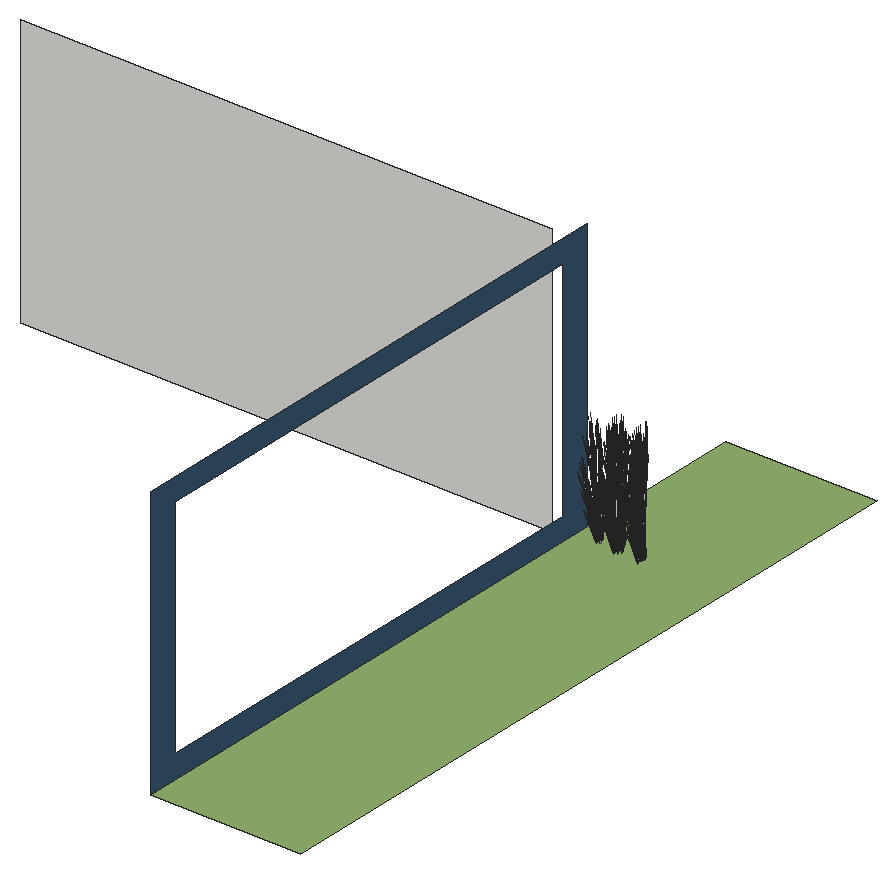
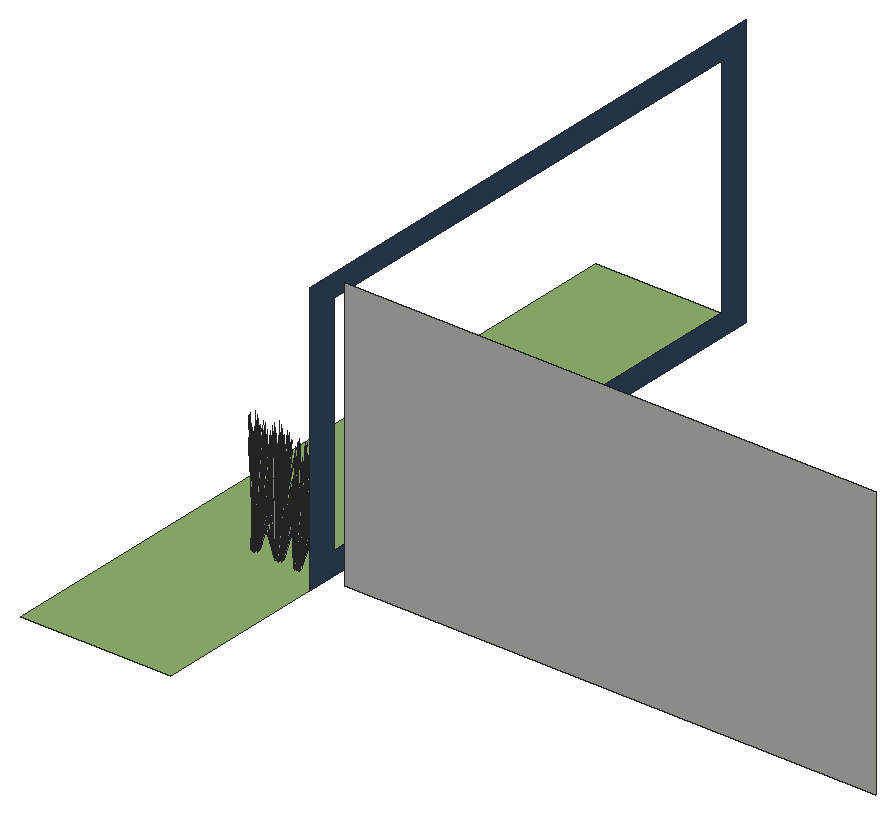
# SketchUp Ruby script. Lengths in inches.
U = 1.inch
M = Sketchup.active_model
def pt(a) = Geom::Point3d.new(a.map { |v| v * U })
def face(e, loops, mat)
  f = e.add_face(loops[0].map { |a| pt(a) })
  loops[1..].each { |l| e.add_face(l.map { |a| pt(a) }).erase! }
  f.material = f.back_material = mat if mat
  f
end
# faces: each face lists its corners as indices into pts; further lists are holes
def faces(e, pts, list, mat = nil) = list.each { |f| face(e, (f[0].is_a?(Array) ? f : [f]).map { |l| l.map { |i| pts[i] } }, mat) }
# xy, xz, yz: faces in a plane at the given z, y or x. An outline is a flat list of corners, or four numbers for a rectangle; further outlines are holes
def ring(l) = l.size == 4 ? [[l[0], l[1]], [l[2], l[1]], [l[2], l[3]], [l[0], l[3]]] : l.each_slice(2).to_a
def flat(e, list, mat, &to3) = list.each { |f| face(e, (f[0].is_a?(Array) ? f : [f]).map { |l| ring(l).map { |u, v| to3.(u, v) } }, mat) }
def xy(e, z, list, mat = nil) = flat(e, list, mat) { |x, y| [x, y, z] }
def xz(e, y, list, mat = nil) = flat(e, list, mat) { |x, z| [x, y, z] }
def yz(e, x, list, mat = nil) = flat(e, list, mat) { |y, z| [x, y, z] }
def lines(e, pts, list) = list.each { |a, b| e.add_line(pt(pts[a]), pt(pts[b])) }
# prism: a flat outline (further loops are holes) pulled along v
def prism(e, loops, v, mat = nil)
  f = face(e, loops, mat); d = Geom::Vector3d.new(v.map { |x| x * U })
  f.pushpull(f.normal.samedirection?(d) ? d.length : -d.length)
end
def box(e, o, s, mat = nil) = prism(e, [[o, [o[0] + s[0], o[1], o[2]], [o[0] + s[0], o[1] + s[1], o[2]], [o[0], o[1] + s[1], o[2]]]], [0, 0, s[2]], mat)
def at(x, y, z, deg = 0) = Geom::Transformation.translation(pt([x, y, z])) * Geom::Transformation.rotation(ORIGIN, Z_AXIS, deg.degrees)
def axes(o, x, y, z) = Geom::Transformation.new([*x, 0, *y, 0, *z, 0, *pt(o).to_a, 1])
def part(name) = M.definitions.add(name)
# library, detail: a bought-in or finely detailed component or shape, given as its bounding box
def library(name, o, s) = part(name).tap { |d| box(d.entities, o, s) }
def detail(e, o, s) = box(e.add_group.entities, o, s)
def put(e, d, t, mat = nil) = e.add_instance(d, t).tap { |i| i.material = mat if mat }
def group(e, t, mat = nil) = e.add_group.tap { |g| g.transformation = t; g.material = mat if mat }.entities
root = M.entities
M.materials.add("Carpet_04_1K").color = [56, 85, 112]
M.materials.add("LightPink_Translucent").color = [144, 107, 117]
M.materials["LightPink_Translucent"].alpha = 0.75
M.materials.add("Roofing_02_1K").color = [146, 178, 111]
c1 = part("blade")
p = [[2.15,0.21,22],[0,0.17,0],[0.09,0.45,0],[2.18,0.31,22],[2.29,0.31,22],[0.38,0.45,0],
  [2.48,0.24,33],[2.49,0.24,33],[2.48,0.22,33]]
faces(c1.entities,p,[[0,1,2,3],[4,5,2,3],[6,3,4,7],[8,0,3,6]])
c2 = part("seeds")
p = [[0.3,-0.1,1.38],[-0.01,-0.03,1.59],[-0.01,-0.03,0.03],[0.14,-0.07,-0.07],[0.29,-0.03,3],[0.15,0.01,3.11]]
faces(c2.entities,p,[[0,1,2,3],[1,0,4,5]],"LightPink_Translucent")
c3 = part("blade with seeds")
put(c3.entities,c1,at(0,0,0))
put(c3.entities,c2,axes([2.4,0.25,30.99],[1.5799,-0.05474,1.17369],[-0.12525,1.92788,0.29478],[-0.07173,-0.02425,1.56792]))
xy(root,0,[[330.57,509.26,410.57,890.67]],"Roofing_02_1K")
xz(root,786.64,[[39.57,0,321.57,144]])
yz(root,330.57,[[[509.26,0,798.7,144],[525.34,12,782.62,132]]],"Carpet_04_1K")
put(root,c3,axes([367.32,786.74,3.875],[0.08068,0.14973,1.71376],[-0.3728,0.12606,0.13857],[-0.08426,-0.23506,0.73262]))
put(root,c3,axes([368.3125,786.86,4.98],[-0.16845,-0.3792,-0.71045],[0.34676,-0.21133,0.08574],[-0.03939,-0.18322,1.00501]))
put(root,c3,axes([367.22,786.35,2.59],[-0.02137,0.15256,1.43002],[-0.31245,0.12771,-0.30754],[-0.07303,-0.19719,0.61141]))
put(root,c3,axes([354.24,787.1,3.875],[0.08068,0.14973,1.71376],[-0.3728,0.12606,0.13857],[-0.08426,-0.23506,0.73262]))
put(root,c3,axes([368.02,786.01,1.49],[-0.0592,0.0168,1.76342],[-0.32738,-0.18913,-0.26939],[0.00549,-0.15776,0.30037]))
put(root,c3,axes([355.69,786.88,2.59],[-0.10032,0.0944,1.43002],[-0.30046,-0.16522,-0.30754],[0.05569,-0.20547,0.61141]))
put(root,c3,axes([355.23,787.21,4.98],[-0.16845,-0.3792,-0.71045],[0.34676,-0.21133,0.08574],[-0.03939,-0.18322,1.00501]))
put(root,c3,axes([354.14,786.7,2.59],[-0.02137,0.15256,1.43002],[-0.31245,0.12771,-0.30754],[-0.07303,-0.19719,0.61141]))
put(root,c3,axes([368.34,786.53,4.53],[0.1064,-0.35863,-0.35414],[0.31043,0.1046,0.4572],[-0.02846,-0.14439,0.87481]))
put(root,c3,axes([354.94,786.37,1.49],[-0.0592,0.0168,1.76342],[-0.32738,-0.18913,-0.26939],[0.00549,-0.15776,0.30037]))
put(root,c3,axes([368.1875,786.78,4.68],[-0.34695,-0.11691,-0.51099],[0.11892,-0.40083,-0.3958],[-0.03181,-0.16138,0.97773]))
put(root,c3,axes([368.4,785.78,2.77],[0.04528,0.27194,1.1486],[-0.25117,-0.15062,0.84392],[0.02703,-0.13924,0.25299]))
put(root,c3,axes([355.93,787.58,4.98],[0.00918,-0.43138,-0.71045],[0.38672,0.02897,0.08574],[0.04081,-0.18275,1.00501]))
put(root,c3,axes([368.9375,787.08,4.68],[-0.25266,-0.31335,-0.51099],[0.2669,-0.27442,-0.3958],[0.03844,-0.15921,0.97773]))
put(root,c3,axes([355.27,786.89,4.53],[0.1064,-0.35863,-0.35414],[0.31043,0.1046,0.4572],[-0.02846,-0.14439,0.87481]))
put(root,c3,axes([355.5,787.36,3.875],[-0.06572,0.16029,1.71376],[-0.27569,-0.33172,0.13857],[0.12437,-0.20675,0.73262]))
put(root,c3,axes([355.11,787.13,4.68],[-0.34695,-0.11691,-0.51099],[0.11892,-0.40083,-0.3958],[-0.03181,-0.16138,0.97773]))
put(root,c3,axes([355.32,786.13,2.77],[0.04528,0.27194,1.1486],[-0.25117,-0.15062,0.84392],[0.02703,-0.13924,0.25299]))
put(root,c3,axes([355.86,787.4375,4.68],[-0.25266,-0.31335,-0.51099],[0.2669,-0.27442,-0.3958],[0.03844,-0.15921,0.97773]))
put(root,c3,axes([367.11,786.1,2.77],[0.18411,0.16231,1.1486],[-0.26813,0.09757,0.84392],[-0.05737,-0.12474,0.25299]))
put(root,c3,axes([367.55,786.96,4.98],[-0.30095,-0.22541,-0.71045],[0.21388,-0.395,0.08574],[-0.10904,-0.13459,1.00501]))
put(root,c3,axes([367.45,786.66,4.53],[-0.05451,-0.37564,-0.35414],[0.31161,-0.09919,0.4572],[-0.0837,-0.10765,0.87481]))
put(root,c3,axes([356.09,787.32,4.53],[0.23881,-0.24554,-0.35414],[0.22606,0.28036,0.4572],[0.0344,-0.14245,0.87481]))
put(root,c3,axes([354.03,786.46,2.77],[0.18411,0.16231,1.1486],[-0.26813,0.09757,0.84392],[-0.05737,-0.12474,0.25299]))
put(root,c3,axes([354.47,787.32,4.98],[-0.30095,-0.22541,-0.71045],[0.21388,-0.395,0.08574],[-0.10904,-0.13459,1.00501]))
put(root,c3,axes([354.37,787.02,4.53],[-0.05451,-0.37564,-0.35414],[0.31161,-0.09919,0.4572],[-0.0837,-0.10765,0.87481]))
put(root,c3,axes([366.96,786.59,1.49],[-0.03419,0.06144,1.76342],[-0.3455,0.13246,-0.26939],[-0.08346,-0.12049,0.30037]))
put(root,c3,axes([367.53,788.28,2.1],[-0.14494,-0.47823,-0.69835],[0.41752,-0.17223,-0.18329],[-0.01602,-0.16194,1.54149]))
put(root,c3,axes([366.78,787.21,3.875],[0.1311,0.08035,1.71376],[-0.27131,0.33708,0.13857],[-0.16909,-0.15206,0.73262]))
put(root,c3,axes([367.41,786.97,4.68],[-0.34827,0.11086,-0.51099],[-0.06092,-0.41983,-0.3958],[-0.09354,-0.12031,0.97773]))
put(root,c3,axes([353.88,786.95,1.49],[-0.03419,0.06144,1.76342],[-0.3455,0.13246,-0.26939],[-0.08346,-0.12049,0.30037]))
put(root,c3,axes([354.45,788.63,2.1],[-0.14494,-0.47823,-0.69835],[0.41752,-0.17223,-0.18329],[-0.01602,-0.16194,1.54149]))
put(root,c3,axes([353.7,787.57,3.875],[0.1311,0.08035,1.71376],[-0.27131,0.33708,0.13857],[-0.16909,-0.15206,0.73262]))
put(root,c3,axes([356.39,787.17,1.49],[-0.05283,-0.03674,1.76342],[-0.13569,-0.41045,-0.26939],[0.09154,-0.11138,0.30037]))
put(root,c3,axes([367.48,786.91,2.375],[-0.22066,-0.46731,0],[0.36918,-0.26061,-0.51607],[0.08408,-0.05936,1.63711]))
put(root,c3,axes([367.96,786.34,2.13],[-0.2439,0.26754,-0.03893],[-0.22348,-0.29302,-0.17649],[-0.01573,-0.08303,0.58215]))
put(root,c3,axes([354.33,787.33,4.68],[-0.34827,0.11086,-0.51099],[-0.06092,-0.41983,-0.3958],[-0.09354,-0.12031,0.97773]))
put(root,c3,axes([356.39,788.33,4.98],[0.18436,-0.36797,-0.71045],[0.32306,0.26151,0.08574],[0.11008,-0.13332,1.00501]))
put(root,c3,axes([354.4,787.26,2.375],[-0.22066,-0.46731,0],[0.36918,-0.26061,-0.51607],[0.08408,-0.05936,1.63711]))
put(root,c3,axes([356.38,788.16,4.68],[-0.09067,-0.42583,-0.51099],[0.34336,-0.07449,-0.3958],[0.0984,-0.11438,0.97773]))
put(root,c3,axes([354.88,786.7,2.13],[-0.2439,0.26754,-0.03893],[-0.22348,-0.29302,-0.17649],[-0.01573,-0.08303,0.58215]))
put(root,c3,axes([368.27,789.51,3.33],[0.305,0.18805,1.51261],[-0.29879,0.40513,0.59816],[-0.13384,-0.24012,1.26806]))
put(root,c3,axes([342.99,789.57,3.875],[0.08068,0.14973,1.71376],[-0.3728,0.12606,0.13857],[-0.08426,-0.23506,0.73262]))
put(root,c3,axes([366.68,788.21,2.02],[0,-0.46636,-0.49651],[0.39487,0,0],[0,-0.10622,1.57504]))
put(root,c3,axes([344.44,789.35,2.59],[-0.10032,0.0944,1.43002],[-0.30046,-0.16522,-0.30754],[0.05569,-0.20547,0.61141]))
put(root,c3,axes([343.98,789.68,4.98],[-0.16845,-0.3792,-0.71045],[0.34676,-0.21133,0.08574],[-0.03939,-0.18322,1.00501]))
put(root,c3,axes([342.89,789.18,2.59],[-0.02137,0.15256,1.43002],[-0.31245,0.12771,-0.30754],[-0.07303,-0.19719,0.61141]))
put(root,c3,axes([355.19,789.87,3.33],[0.305,0.18805,1.51261],[-0.29879,0.40513,0.59816],[-0.13384,-0.24012,1.26806]))
put(root,c3,axes([343.69,788.84,1.49],[-0.0592,0.0168,1.76342],[-0.32738,-0.18913,-0.26939],[0.00549,-0.15776,0.30037]))
put(root,c3,axes([353.6,788.57,2.02],[0,-0.46636,-0.49651],[0.39487,0,0],[0,-0.10622,1.57504]))
put(root,c3,axes([354.7,787.1875,2.02],[0.33032,-0.23318,-0.49651],[0.19744,0.41812,0],[0.07523,-0.05311,1.57504]))
put(root,c3,axes([356.66,787.99,2.59],[-0.12609,-0.01381,1.43002],[-0.12917,-0.37055,-0.30754],[0.1549,-0.10482,0.61141]))
put(root,c3,axes([367.75,788.4,2.21],[0.17124,-0.42022,-0.44739],[0.35581,0.20224,0.21531],[0,-0.09687,1.43643]))
put(root,c3,axes([366.73,787.33,4.53],[-0.20082,-0.29199,-0.35414],[0.2293,-0.2764,0.4572],[-0.1165,-0.04206,0.87481]))
put(root,c3,axes([355.09,788.14,2.06],[0.23773,-0.35053,-0.62353],[0.29532,0.31785,-0.16365],[0.09526,-0.08744,1.37633]))
put(root,c3,axes([344.68,790.05,4.98],[0.00918,-0.43138,-0.71045],[0.38672,0.02897,0.08574],[0.04081,-0.18275,1.00501]))
put(root,c3,axes([367.91,788.2,2.67],[-0.04113,-0.53214,-0.29095],[0.42835,-0.03218,-0.50002],[0.07543,-0.07088,1.59708]))
put(root,c3,axes([356.8,787.3125,2.77],[-0.11756,0.2374,1.1486],[-0.10105,-0.31895,0.84392],[0.09709,-0.07992,0.25299]))
put(root,c3,axes([366.85,788.22,2.03],[0.24637,-0.29097,-0.30978],[0.24637,0.29097,0.30978],[0,-0.09372,1.38974]))
put(root,c3,axes([366.75,786.83,2.13],[-0.10181,0.3808,-0.03893],[-0.31336,-0.11714,-0.17649],[-0.04758,-0.06228,0.58215]))
put(root,c3,axes([367.71,788.75,2.67],[-0.39748,-0.22252,-0.29095],[0.19139,-0.46966,-0.50002],[-0.01249,-0.11531,1.59708]))
put(root,c3,axes([344.01,789.36,4.53],[0.1064,-0.35863,-0.35414],[0.31043,0.1046,0.4572],[-0.02846,-0.14439,0.87481]))
put(root,c3,axes([344.25,789.83,3.875],[-0.06572,0.16029,1.71376],[-0.27569,-0.33172,0.13857],[0.12437,-0.20675,0.73262]))
put(root,c3,axes([366.58,788.57,2.375],[-0.44133,0,0],[0,-0.52122,-0.51607],[0,-0.11871,1.63711]))
put(root,c3,axes([356.63,788.2,4.53],[0.30722,-0.06665,-0.35414],[0.08112,0.381,0.4572],[0.08804,-0.10234,0.87481]))
put(root,c3,axes([366.66,787.64,2.59],[0.06891,0.12984,1.43002],[-0.15879,0.35293,-0.30754],[-0.16304,-0.08436,0.61141]))
put(root,c3,axes([343.86,789.61,4.68],[-0.34695,-0.11691,-0.51099],[0.11892,-0.40083,-0.3958],[-0.03181,-0.16138,0.97773]))
put(root,c3,axes([354.67,788.76,2.21],[0.17124,-0.42022,-0.44739],[0.35581,0.20224,0.21531],[0,-0.09687,1.43643]))
put(root,c3,axes([353.65,787.68,4.53],[-0.20082,-0.29199,-0.35414],[0.2293,-0.2764,0.4572],[-0.1165,-0.04206,0.87481]))
put(root,c3,axes([344.07,788.6,2.77],[0.04528,0.27194,1.1486],[-0.25117,-0.15062,0.84392],[0.02703,-0.13924,0.25299]))
put(root,c3,axes([354.83,788.55,2.67],[-0.04113,-0.53214,-0.29095],[0.42835,-0.03218,-0.50002],[0.07543,-0.07088,1.59708]))
put(root,c3,axes([366.94,787.52,4.98],[-0.35281,-0.01123,-0.71045],[0.0237,-0.47284,0.08574],[-0.14947,-0.0499,1.00501]))
put(root,c3,axes([344.61,789.91,4.68],[-0.25266,-0.31335,-0.51099],[0.2669,-0.27442,-0.3958],[0.03844,-0.15921,0.97773]))
put(root,c3,axes([353.77,788.58,2.03],[0.24637,-0.29097,-0.30978],[0.24637,0.29097,0.30978],[0,-0.09372,1.38974]))
put(root,c3,axes([353.67,787.18,2.13],[-0.10181,0.3808,-0.03893],[-0.31336,-0.11714,-0.17649],[-0.04758,-0.06228,0.58215]))
put(root,c3,axes([354.63,789.11,2.67],[-0.39748,-0.22252,-0.29095],[0.19139,-0.46966,-0.50002],[-0.01249,-0.11531,1.59708]))
put(root,c3,axes([353.5,788.92,2.375],[-0.44133,0,0],[0,-0.52122,-0.51607],[0,-0.11871,1.63711]))
put(root,c3,axes([353.58,787.99,2.59],[0.06891,0.12984,1.43002],[-0.15879,0.35293,-0.30754],[-0.16304,-0.08436,0.61141]))
put(root,c3,axes([354.77,787.37,2.03],[0.32928,0.11539,-0.30978],[-0.08291,0.40636,0.30978],[0.06638,-0.04686,1.38974]))
put(root,c3,axes([353.86,787.875,4.98],[-0.35281,-0.01123,-0.71045],[0.0237,-0.47284,0.08574],[-0.14947,-0.0499,1.00501]))
put(root,c3,axes([366.92,788.43,2.33],[-0.32829,0.39208,0.30756],[-0.32849,-0.38796,-0.36492],[-0.01146,-0.11134,1.64885]))
put(root,c3,axes([344.84,789.79,4.53],[0.23881,-0.24554,-0.35414],[0.22606,0.28036,0.4572],[0.0344,-0.14245,0.87481]))
put(root,c3,axes([342.78,788.93,2.77],[0.18411,0.16231,1.1486],[-0.26813,0.09757,0.84392],[-0.05737,-0.12474,0.25299]))
put(root,c3,axes([343.22,789.79,4.98],[-0.30095,-0.22541,-0.71045],[0.21388,-0.395,0.08574],[-0.10904,-0.13459,1.00501]))
put(root,c3,axes([343.12,789.49,4.53],[-0.05451,-0.37564,-0.35414],[0.31161,-0.09919,0.4572],[-0.0837,-0.10765,0.87481]))
put(root,c3,axes([367.97,788.61,2.43],[0.39767,0.22603,0.24065],[-0.19139,0.46966,0.50002],[0,-0.10827,1.60543]))
put(root,c3,axes([367.8125,789.25,2.4375],[0.09355,-0.55261,-0.23429],[0.44354,0.09633,0.51271],[-0.0775,-0.07631,1.5644]))
put(root,c3,axes([366.82,787.62,4.68],[-0.25628,0.30892,-0.51099],[-0.22444,-0.32634,-0.3958],[-0.13021,-0.047,0.97773]))
put(root,c3,axes([366.25,788.03,2.77],[0.22533,-0.03337,1.1486],[-0.14293,0.29403,0.84392],[-0.11135,-0.04411,0.25299]))
put(root,c3,axes([353.84,788.78,2.33],[-0.32829,0.39208,0.30756],[-0.32849,-0.38796,-0.36492],[-0.01146,-0.11134,1.64885]))
put(root,c3,axes([342.63,789.42,1.49],[-0.03419,0.06144,1.76342],[-0.3455,0.13246,-0.26939],[-0.08346,-0.12049,0.30037]))
put(root,c3,axes([367.84,788.3,2.72],[-0.38326,0.02879,0.44739],[-0.03466,-0.47788,-0.21531],[0.06861,-0.04843,1.43643]))
put(root,c3,axes([366.85,788.65,2.48],[0,0.46636,0.49651],[-0.39487,0,0],[0,-0.10622,1.57504]))
put(root,c3,axes([354.89,788.97,2.43],[0.39767,0.22603,0.24065],[-0.19139,0.46966,0.50002],[0,-0.10827,1.60543]))
put(root,c3,axes([354.73,789.6,2.4375],[0.09355,-0.55261,-0.23429],[0.44354,0.09633,0.51271],[-0.0775,-0.07631,1.5644]))
put(root,c3,axes([343.2,791.11,2.1],[-0.14494,-0.47823,-0.69835],[0.41752,-0.17223,-0.18329],[-0.01602,-0.16194,1.54149]))
put(root,c3,axes([342.45,790.04,3.875],[0.1311,0.08035,1.71376],[-0.27131,0.33708,0.13857],[-0.16909,-0.15206,0.73262]))
put(root,c3,axes([345.14,789.65,1.49],[-0.05283,-0.03674,1.76342],[-0.13569,-0.41045,-0.26939],[0.09154,-0.11138,0.30037]))
put(root,c3,axes([353.74,787.97,4.68],[-0.25628,0.30892,-0.51099],[-0.22444,-0.32634,-0.3958],[-0.13021,-0.047,0.97773]))
put(root,c3,axes([366.5,787.95,3.875],[0.14639,-0.01056,1.71376],[-0.09712,0.45778,0.13857],[-0.20862,-0.02831,0.73262]))
put(root,c3,axes([367.78,789.02,2.21],[-0.21202,-0.39143,-0.44739],[0.32115,-0.27564,0.21531],[-0.06861,-0.04843,1.43643]))
put(root,c3,axes([367.83,788.47,2.36],[0.15345,0.52148,0.45755],[-0.43845,0.18134,0.17955],[0.00536,-0.09582,1.58856]))
put(root,c3,axes([353.17,788.38,2.77],[0.22533,-0.03337,1.1486],[-0.14293,0.29403,0.84392],[-0.11135,-0.04411,0.25299]))
put(root,c3,axes([367.75,788.88,2.72],[-0.17124,0.42022,0.44739],[-0.35581,-0.20224,-0.21531],[0,-0.09687,1.43643]))
put(root,c3,axes([343.08,789.8,4.68],[-0.34827,0.11086,-0.51099],[-0.06092,-0.41983,-0.3958],[-0.09354,-0.12031,0.97773]))
put(root,c3,axes([354.76,788.65,2.72],[-0.38326,0.02879,0.44739],[-0.03466,-0.47788,-0.21531],[0.06861,-0.04843,1.43643]))
put(root,c3,axes([368.375,788.51,2.21],[0,-0.53961,0],[0.44133,0,0],[0,0,1.79456]))
put(root,c3,axes([353.77,789,2.48],[0,0.46636,0.49651],[-0.39487,0,0],[0,-0.10622,1.57504]))
put(root,c3,axes([356.54,789.1,4.68],[0.09562,-0.42421,-0.51099],[0.32782,0.1454,-0.3958],[0.13199,-0.0389,0.97773]))
put(root,c3,axes([356.02,787.38,2.375],[0.22066,-0.46731,0],[0.36918,0.26061,-0.51607],[0.08408,0.05936,1.63711]))
put(root,c3,axes([353.42,788.3,3.875],[0.14639,-0.01056,1.71376],[-0.09712,0.45778,0.13857],[-0.20862,-0.02831,0.73262]))
put(root,c3,axes([354.7,789.375,2.21],[-0.21202,-0.39143,-0.44739],[0.32115,-0.27564,0.21531],[-0.06861,-0.04843,1.43643]))
put(root,c3,axes([354.75,788.82,2.36],[0.15345,0.52148,0.45755],[-0.43845,0.18134,0.17955],[0.00536,-0.09582,1.58856]))
put(root,c3,axes([345.14,790.8,4.98],[0.18436,-0.36797,-0.71045],[0.32306,0.26151,0.08574],[0.11008,-0.13332,1.00501]))
put(root,c3,axes([343.15,789.73,2.375],[-0.22066,-0.46731,0],[0.36918,-0.26061,-0.51607],[0.08408,-0.05936,1.63711]))
put(root,c3,axes([367.59,789.17,2.06],[-0.36714,-0.07646,-0.62353],[0.07747,-0.47163,-0.16365],[-0.10956,-0.05715,1.37633]))
put(root,c3,axes([345.13,790.63,4.68],[-0.09067,-0.42583,-0.51099],[0.34336,-0.07449,-0.3958],[0.0984,-0.11438,0.97773]))
put(root,c3,axes([368.17,788.17,2.36],[-0.29264,0.42323,0.45755],[-0.34767,-0.3736,0.17955],[0.07055,-0.04224,1.58856]))
put(root,c3,axes([343.63,789.17,2.13],[-0.2439,0.26754,-0.03893],[-0.22348,-0.29302,-0.17649],[-0.01573,-0.08303,0.58215]))
put(root,c3,axes([356.89,789.22,1.98],[-0.22732,0.05597,1.41583],[-0.03618,-0.44548,0.08104],[0.15921,-0.06743,0.80566]))
put(root,c3,axes([357.31,788.83,2.26],[-0.21881,-0.29821,-0.06488],[0.23965,-0.27324,-0.29416],[0.0679,-0.01924,0.97024]))
put(root,c3,axes([368.49,788.93,2.3],[-0.32829,-0.4014,-0.06131],[0.32849,-0.40164,0],[-0.01146,-0.01402,1.75571]))
put(root,c3,axes([354.67,789.23,2.72],[-0.17124,0.42022,0.44739],[-0.35581,-0.20224,-0.21531],[0,-0.09687,1.43643]))
put(root,c3,axes([367.66,787.48,2.47],[-0.10196,0.46348,0.17642],[-0.3731,-0.13116,0.35086],[0.06445,-0.00226,1.60407]))
put(root,c3,axes([355.3,788.87,2.21],[0,-0.53961,0],[0.44133,0,0],[0,0,1.79456]))
put(root,c3,axes([355.83,787.62,2.48],[-0.33032,-0.23318,0.49651],[0.19744,-0.41812,0],[0.07523,0.05311,1.57504]))
put(root,c3,axes([356.48,789.26,4.98],[0.31014,-0.20596,-0.71045],[0.17284,0.42397,0.08574],[0.14985,-0.04816,1.00501]))
put(root,c3,axes([367.86,788.98,2.36],[0.44609,0.09826,0.45755],[-0.09078,0.55493,0.17955],[-0.06519,-0.05359,1.58856]))
put(root,c3,axes([354.51,789.53,2.06],[-0.36714,-0.07646,-0.62353],[0.07747,-0.47163,-0.16365],[-0.10956,-0.05715,1.37633]))
put(root,c3,axes([355.09,788.53,2.36],[-0.29264,0.42323,0.45755],[-0.34767,-0.3736,0.17955],[0.07055,-0.04224,1.58856]))
put(root,c3,axes([366.41,788.51,1.49],[0.00895,0.0735,1.76342],[-0.18044,0.38382,-0.26939],[-0.12817,-0.01935,0.30037]))
put(root,c3,axes([343.94,792.34,3.33],[0.305,0.18805,1.51261],[-0.29879,0.40513,0.59816],[-0.13384,-0.24012,1.26806]))
put(root,c3,axes([368.3,788.1,2.72],[-0.21202,-0.39143,0.44739],[0.32115,-0.27564,-0.21531],[0.06861,0.04843,1.43643]))
put(root,c3,axes([355.41,789.29,2.3],[-0.32829,-0.4014,-0.06131],[0.32849,-0.40164,0],[-0.01146,-0.01402,1.75571]))
put(root,c3,axes([354.58,787.83,2.47],[-0.10196,0.46348,0.17642],[-0.3731,-0.13116,0.35086],[0.06445,-0.00226,1.60407]))
put(root,c3,axes([367.2,789.89,2.03],[-0.08291,-0.40636,-0.30978],[0.32928,-0.11539,0.30978],[-0.06638,-0.04686,1.38974]))
put(root,c3,axes([342.35,791.04,2.02],[0,-0.46636,-0.49651],[0.39487,0,0],[0,-0.10622,1.57504]))
put(root,c3,axes([343.45,789.66,2.02],[0.33032,-0.23318,-0.49651],[0.19744,0.41812,0],[0.07523,-0.05311,1.57504]))
put(root,c3,axes([345.41,790.47,2.59],[-0.12609,-0.01381,1.43002],[-0.12917,-0.37055,-0.30754],[0.1549,-0.10482,0.61141]))
put(root,c3,axes([354.43,788.21,1.59],[-0.3474,0.18671,1.28929],[-0.11057,-0.53572,0.50096],[0.21332,0.00891,1.46642]))
put(root,c3,axes([355.36,788.35,2.62],[0.06809,-0.4162,0.1448],[0.33266,0.07225,-0.41347],[0.06054,0.04274,1.26744]))
put(root,c3,axes([367.625,789.87,2.47],[0.37926,-0.12378,0.17642],[0.09365,0.46065,0.35086],[-0.03382,-0.06712,1.60407]))
put(root,c3,axes([343.84,790.62,2.06],[0.23773,-0.35053,-0.62353],[0.29532,0.31785,-0.16365],[0.09526,-0.08744,1.37633]))
put(root,c3,axes([345.55,789.78,2.77],[-0.11756,0.2374,1.1486],[-0.10105,-0.31895,0.84392],[0.09709,-0.07992,0.25299]))
put(root,c3,axes([354.78,789.34,2.36],[0.44609,0.09826,0.45755],[-0.09078,0.55493,0.17955],[-0.06519,-0.05359,1.58856]))
put(root,c3,axes([357.14,788.93,1.49],[-0.01845,-0.0708,1.76342],[0.12793,-0.41416,-0.26939],[0.12905,-0.00596,0.30037]))
put(root,c3,axes([367.11,790.07,2.02],[-0.33032,-0.23318,-0.49651],[0.19744,-0.41812,0],[-0.07523,-0.05311,1.57504]))
put(root,c3,axes([353.33,788.86,1.49],[0.00895,0.0735,1.76342],[-0.18044,0.38382,-0.26939],[-0.12817,-0.01935,0.30037]))
put(root,c3,axes([366.375,788.34,4.53],[-0.29332,-0.1301,-0.35414],[0.08555,-0.37955,0.4572],[-0.11809,0.0348,0.87481]))
put(root,c3,axes([355.22,788.46,2.72],[-0.21202,-0.39143,0.44739],[0.32115,-0.27564,-0.21531],[0.06861,0.04843,1.43643]))
put(root,c3,axes([368.68,788.63,2.21],[0.39487,0,0],[0,0.48281,0],[0,0,1.78407]))
put(root,c3,axes([354.12,790.25,2.03],[-0.08291,-0.40636,-0.30978],[0.32928,-0.11539,0.30978],[-0.06638,-0.04686,1.38974]))
put(root,c3,axes([368.01,789.24,2.67],[-0.35635,0.30962,-0.29095],[-0.23697,-0.43749,-0.50002],[-0.08792,-0.04443,1.59708]))
put(root,c3,axes([368.79,787.5,2.47],[-0.37926,0.12378,0.17642],[-0.09365,-0.46065,0.35086],[0.03382,0.06712,1.60407]))
put(root,c3,axes([345.38,790.68,4.53],[0.30722,-0.06665,-0.35414],[0.08112,0.381,0.4572],[0.08804,-0.10234,0.87481]))
put(root,c3,axes([343.42,791.23,2.21],[0.17124,-0.42022,-0.44739],[0.35581,0.20224,0.21531],[0,-0.09687,1.43643]))
put(root,c3,axes([342.4,790.15,4.53],[-0.20082,-0.29199,-0.35414],[0.2293,-0.2764,0.4572],[-0.1165,-0.04206,0.87481]))
put(root,c3,axes([354.54,790.22,2.47],[0.37926,-0.12378,0.17642],[0.09365,0.46065,0.35086],[-0.03382,-0.06712,1.60407]))
put(root,c3,axes([355.33,788.48,2.67],[0.35635,-0.30962,-0.29095],[0.23697,0.43749,-0.50002],[0.08792,0.04443,1.59708]))
put(root,c3,axes([356.74,789.3,4.53],[0.29332,0.1301,-0.35414],[-0.08555,0.37955,0.4572],[0.11809,-0.0348,0.87481]))
put(root,c3,axes([343.58,791.02,2.67],[-0.04113,-0.53214,-0.29095],[0.42835,-0.03218,-0.50002],[0.07543,-0.07088,1.59708]))
put(root,c3,axes([342.52,791.05,2.03],[0.24637,-0.29097,-0.30978],[0.24637,0.29097,0.30978],[0,-0.09372,1.38974]))
put(root,c3,axes([354.03,790.42,2.02],[-0.33032,-0.23318,-0.49651],[0.19744,-0.41812,0],[-0.07523,-0.05311,1.57504]))
put(root,c3,axes([356.22,787.66,2.02],[0.33032,0.23318,-0.49651],[-0.19744,0.41812,0],[0.07523,0.05311,1.57504]))
put(root,c3,axes([342.42,789.66,2.13],[-0.10181,0.3808,-0.03893],[-0.31336,-0.11714,-0.17649],[-0.04758,-0.06228,0.58215]))
put(root,c3,axes([353.29,788.69,4.53],[-0.29332,-0.1301,-0.35414],[0.08555,-0.37955,0.4572],[-0.11809,0.0348,0.87481]))
put(root,c3,axes([343.38,791.58,2.67],[-0.39748,-0.22252,-0.29095],[0.19139,-0.46966,-0.50002],[-0.01249,-0.11531,1.59708]))
put(root,c3,axes([355.6,788.99,2.21],[0.39487,0,0],[0,0.48281,0],[0,0,1.78407]))
put(root,c3,axes([368.55,788.39,2.38],[-0.44609,-0.09826,0.49198],[0.09078,-0.55493,0.19306],[0.06519,0.05359,1.70813]))
put(root,c3,axes([342.25,791.39,2.375],[-0.44133,0,0],[0,-0.52122,-0.51607],[0,-0.11871,1.63711]))
put(root,c3,axes([354.93,789.6,2.67],[-0.35635,0.30962,-0.29095],[-0.23697,-0.43749,-0.50002],[-0.08792,-0.04443,1.59708]))
put(root,c3,axes([368.19,789.76,2.2],[-0.11516,-0.40207,0],[0.32884,-0.1408,0],[0,0,1.54371]))
put(root,c3,axes([355.71,787.86,2.47],[-0.37926,0.12378,0.17642],[-0.09365,-0.46065,0.35086],[0.03382,0.06712,1.60407]))
put(root,c3,axes([367.97,789.38,2.62],[-0.06809,0.4162,0.1448],[-0.33266,-0.07225,-0.41347],[-0.06054,-0.04274,1.26744]))
put(root,c3,axes([342.33,790.46,2.59],[0.06891,0.12984,1.43002],[-0.15879,0.35293,-0.30754],[-0.16304,-0.08436,0.61141]))
put(root,c3,axes([343.52,789.84,2.03],[0.32928,0.11539,-0.30978],[-0.08291,0.40636,0.30978],[0.06638,-0.04686,1.38974]))
put(root,c3,axes([355.94,788.83,3.875],[-0.14639,0.01056,1.71376],[0.09712,-0.45778,0.13857],[0.20862,0.02831,0.73262]))
put(root,c3,axes([356.13,787.83,2.03],[0.08291,0.40636,-0.30978],[-0.32928,0.11539,0.30978],[0.06638,0.04686,1.38974]))
put(root,c3,axes([368.75,789.89,2.47],[0.10196,-0.46348,0.17642],[0.3731,0.13116,0.35086],[-0.06445,0.00226,1.60407]))
put(root,c3,axes([342.61,790.35,4.98],[-0.35281,-0.01123,-0.71045],[0.0237,-0.47284,0.08574],[-0.14947,-0.0499,1.00501]))
put(root,c3,axes([368.67,788.84,2.21],[0.24637,0.30123,0],[-0.24637,0.30123,0],[0,0,1.69266]))
put(root,c3,axes([367.27,788.28,3.34],[0.10032,-0.06746,1.77064],[0.0346,0.47103,0.13857],[-0.2173,0.0625,0.63284]))
put(root,c3,axes([369.33,788.71,2.47],[-0.2773,-0.3397,0.17642],[0.27945,-0.32949,0.35086],[-0.03063,0.06937,1.60407]))
put(root,c3,axes([355.47,788.74,2.38],[-0.44609,-0.09826,0.49198],[0.09078,-0.55493,0.19306],[0.06519,0.05359,1.70813]))
put(root,c3,axes([355.11,790.11,2.2],[-0.11516,-0.40207,0],[0.32884,-0.1408,0],[0,0,1.54371]))
put(root,c3,axes([354.89,789.73,2.62],[-0.06809,0.4162,0.1448],[-0.33266,-0.07225,-0.41347],[-0.06054,-0.04274,1.26744]))
put(root,c3,axes([368.11,789.94,2.2],[-0.35581,-0.20937,0],[0.17124,-0.43505,0],[0,0,1.62707]))
put(root,c3,axes([368.41,789.38,2.46],[-0.34464,-0.37536,-0.25192],[0.29,-0.42149,0.5513],[-0.0928,0.04391,1.68216]))
put(root,c3,axes([367.5,790.1,2.48],[0.33032,0.23318,0.49651],[-0.19744,0.41812,0],[-0.07523,-0.05311,1.57504]))
put(root,c3,axes([355.54,790.06,2.18],[0.37054,-0.15823,-0.19198],[0.1302,0.45581,0.00008],[0.0409,-0.01749,1.73897]))
put(root,c3,axes([355.67,790.25,2.47],[0.10196,-0.46348,0.17642],[0.3731,0.13116,0.35086],[-0.06445,0.00226,1.60407]))
put(root,c3,axes([368.66,788.49,2.72],[0.17124,-0.42022,0.44739],[0.35581,0.20224,-0.21531],[0,0.09687,1.43643]))
put(root,c3,axes([355.59,789.2,2.21],[0.24637,0.30123,0],[-0.24637,0.30123,0],[0,0,1.69266]))
put(root,c3,axes([342.59,791.26,2.33],[-0.32829,0.39208,0.30756],[-0.32849,-0.38796,-0.36492],[-0.01146,-0.11134,1.64885]))
put(root,c3,axes([354.1875,788.63,3.34],[0.10032,-0.06746,1.77064],[0.0346,0.47103,0.13857],[-0.2173,0.0625,0.63284]))
put(root,c3,axes([356.26,789.06,2.47],[-0.2773,-0.3397,0.17642],[0.27945,-0.32949,0.35086],[-0.03063,0.06937,1.60407]))
put(root,c3,axes([355.74,788.55,2.06],[0.36714,0.07646,-0.62353],[-0.07747,0.47163,-0.16365],[0.10956,0.05715,1.37633]))
put(root,c3,axes([368.6,788.73,2.29],[0,0.53934,-0.05637],[-0.44133,0,0],[0,0.01695,1.79368]))
put(root,c3,axes([357.36,789.375,2.77],[-0.21807,0.07699,1.1486],[0.10265,-0.31819,0.84392],[0.11568,0.02177,0.25299]))
put(root,c3,axes([366.57,788.53,4.68],[-0.09562,0.42421,-0.51099],[-0.32782,-0.1454,-0.3958],[-0.13199,0.0389,0.97773]))
put(root,c3,axes([367.31,790.35,2.375],[-0.22066,0.46731,0],[-0.36918,-0.26061,-0.51607],[-0.08408,-0.05936,1.63711]))
put(root,c3,axes([343.64,791.4375,2.43],[0.39767,0.22603,0.24065],[-0.19139,0.46966,0.50002],[0,-0.10827,1.60543]))
put(root,c3,axes([355.03,790.3,2.2],[-0.35581,-0.20937,0],[0.17124,-0.43505,0],[0,0,1.62707]))
put(root,c3,axes([355.33,789.74,2.46],[-0.34464,-0.37536,-0.25192],[0.29,-0.42149,0.5513],[-0.0928,0.04391,1.68216]))
put(root,c3,axes([343.48,792.07,2.4375],[0.09355,-0.55261,-0.23429],[0.44354,0.09633,0.51271],[-0.0775,-0.07631,1.5644]))
put(root,c3,axes([354.42,790.46,2.48],[0.33032,0.23318,0.49651],[-0.19744,0.41812,0],[-0.07523,-0.05311,1.57504]))
